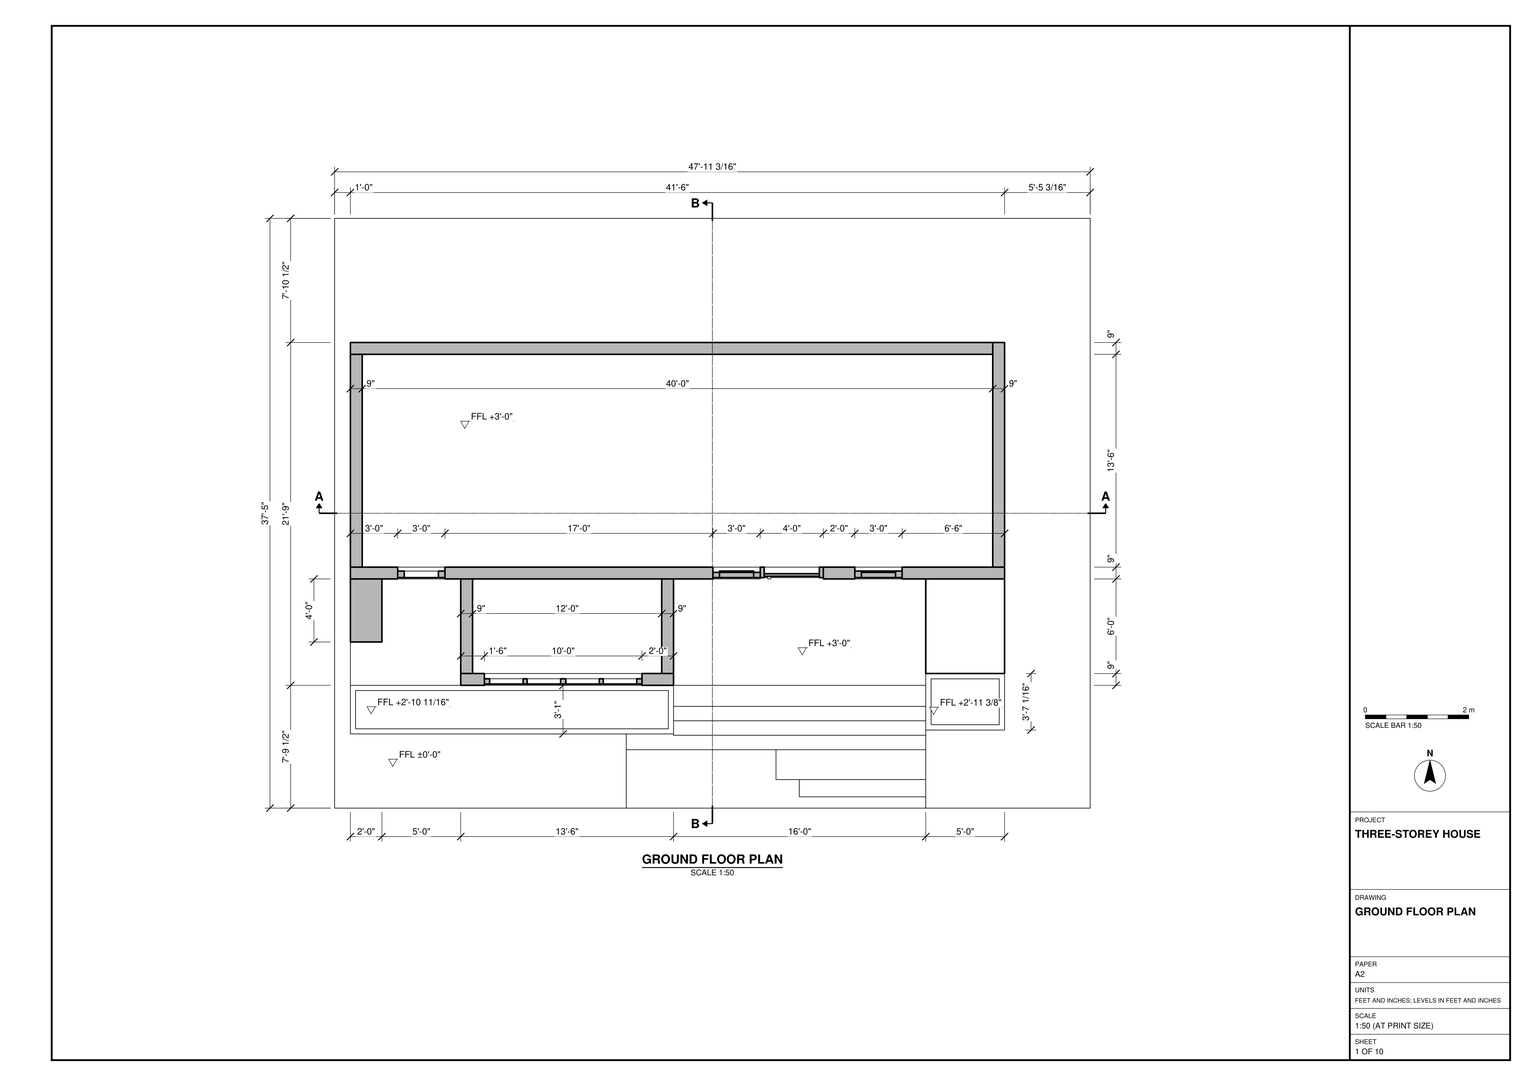
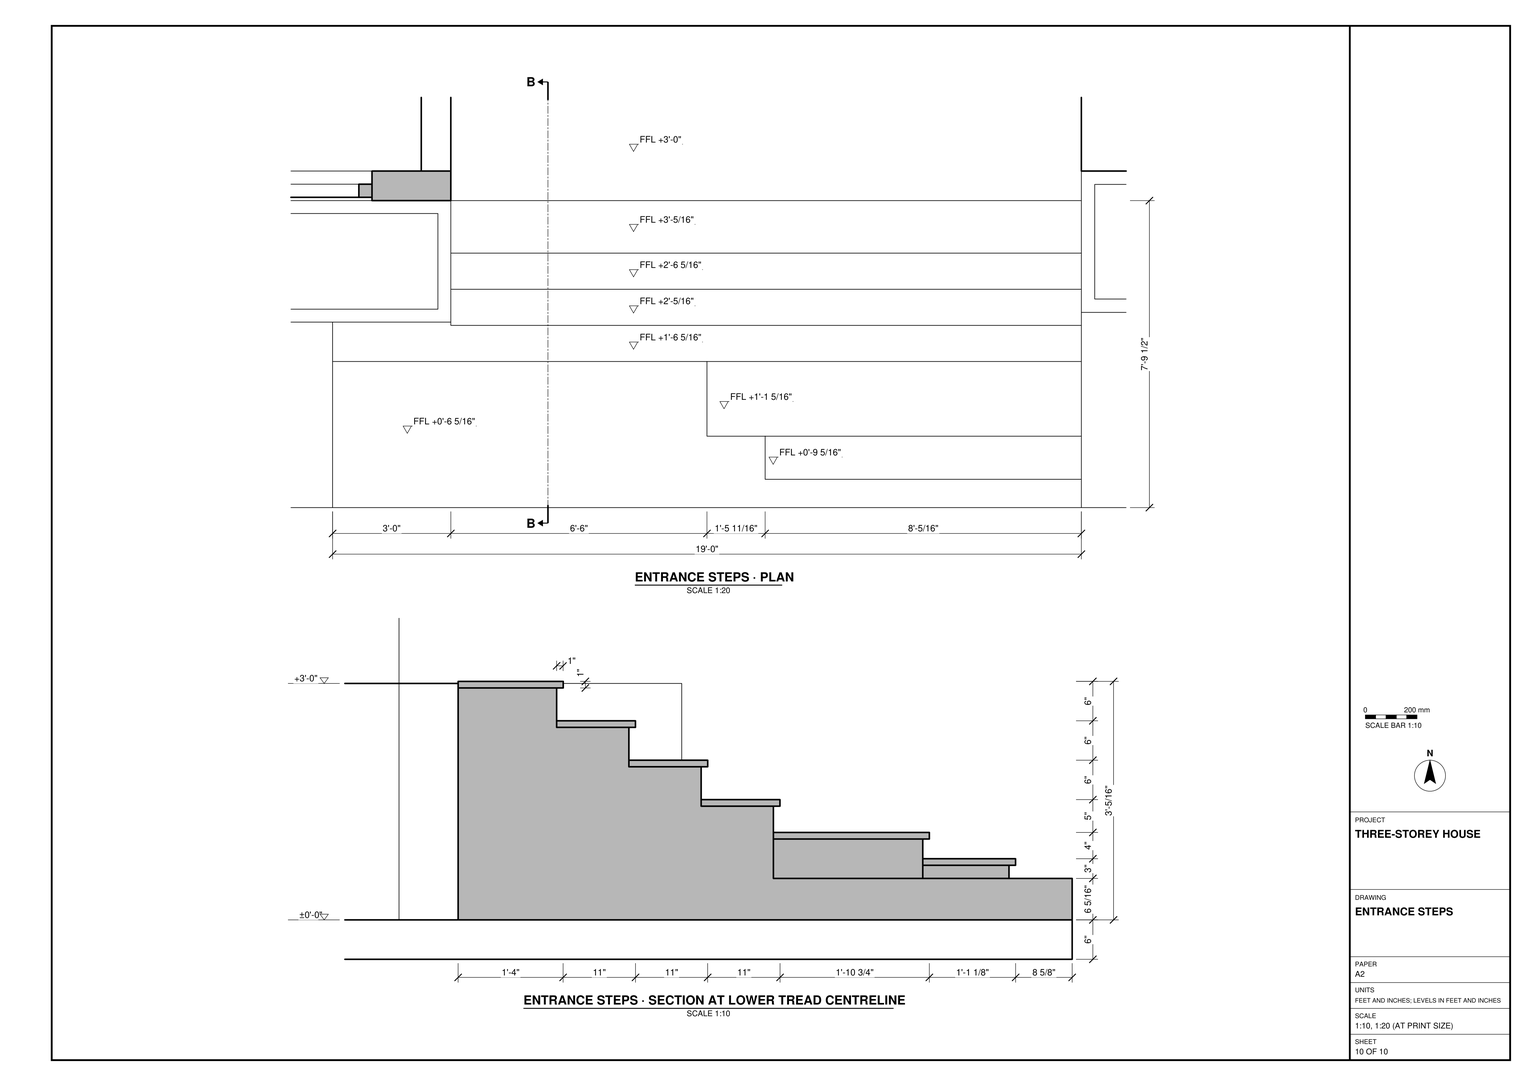
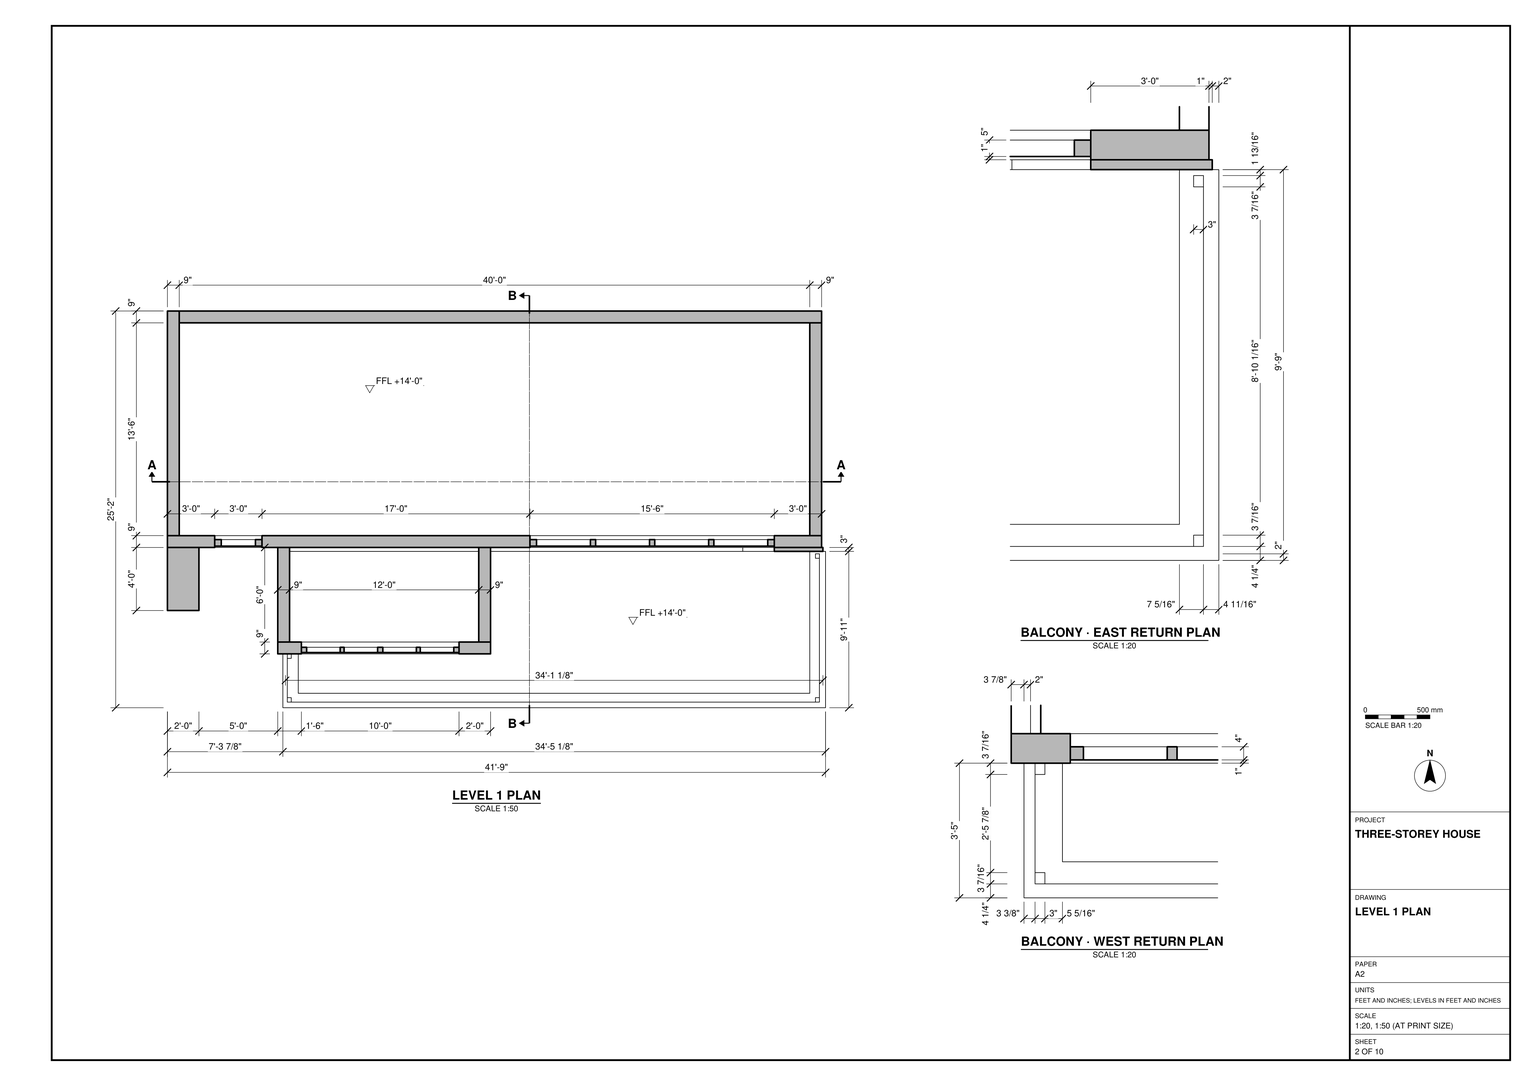
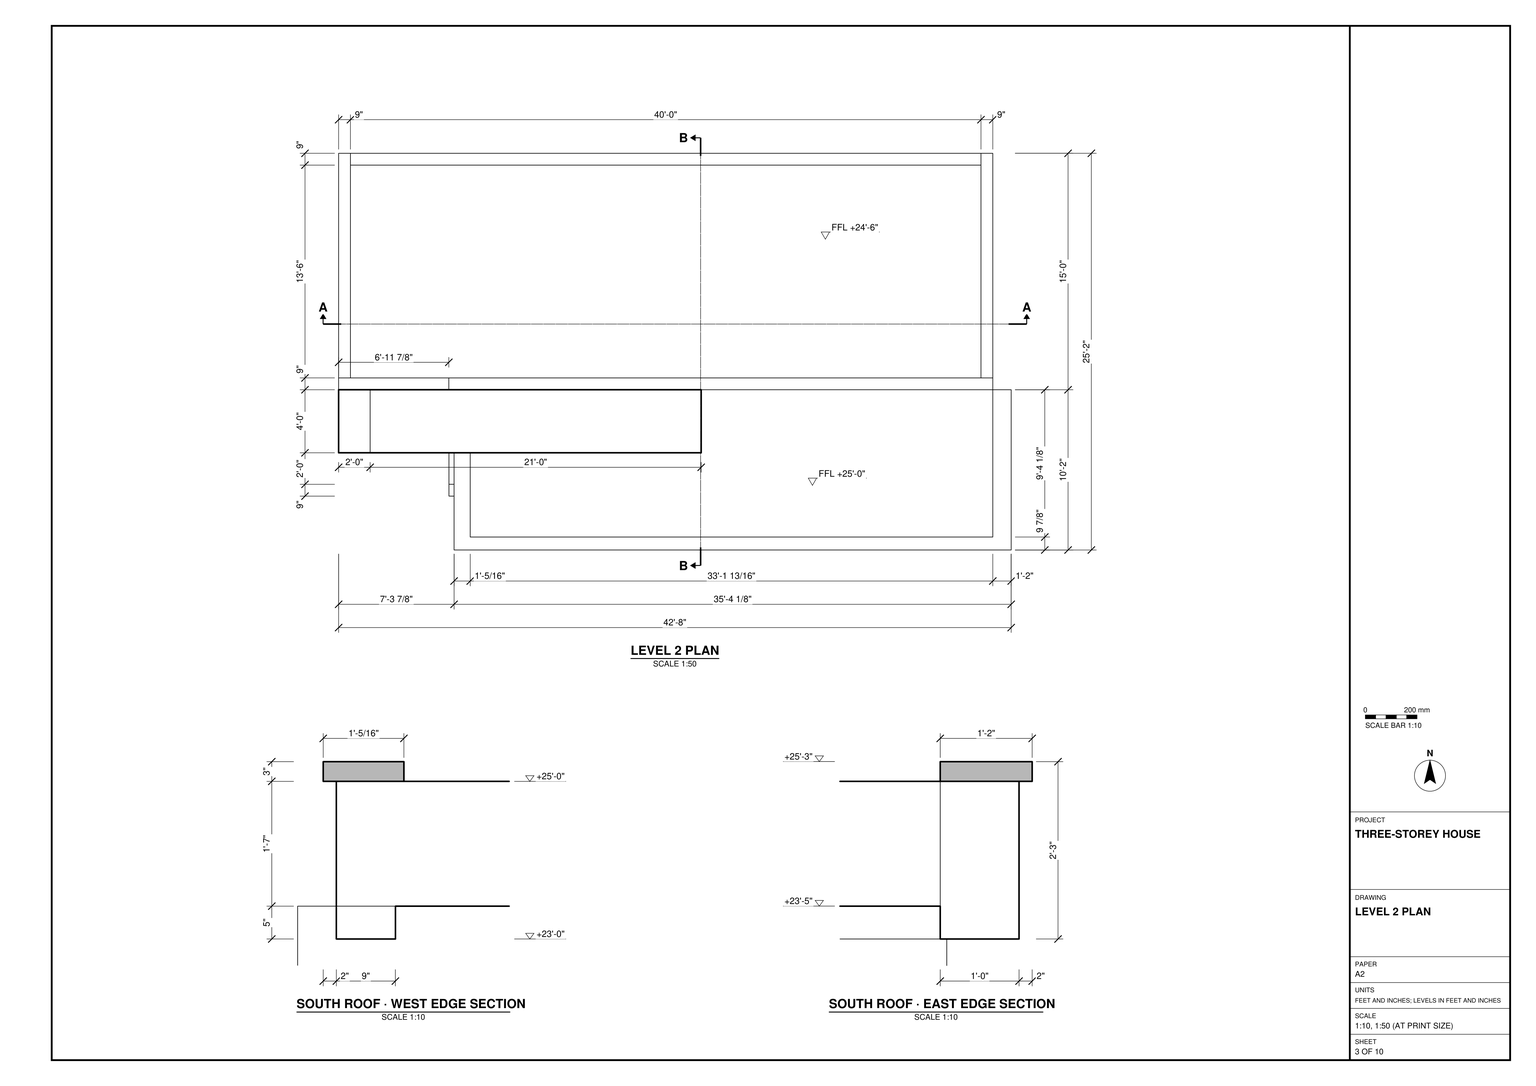
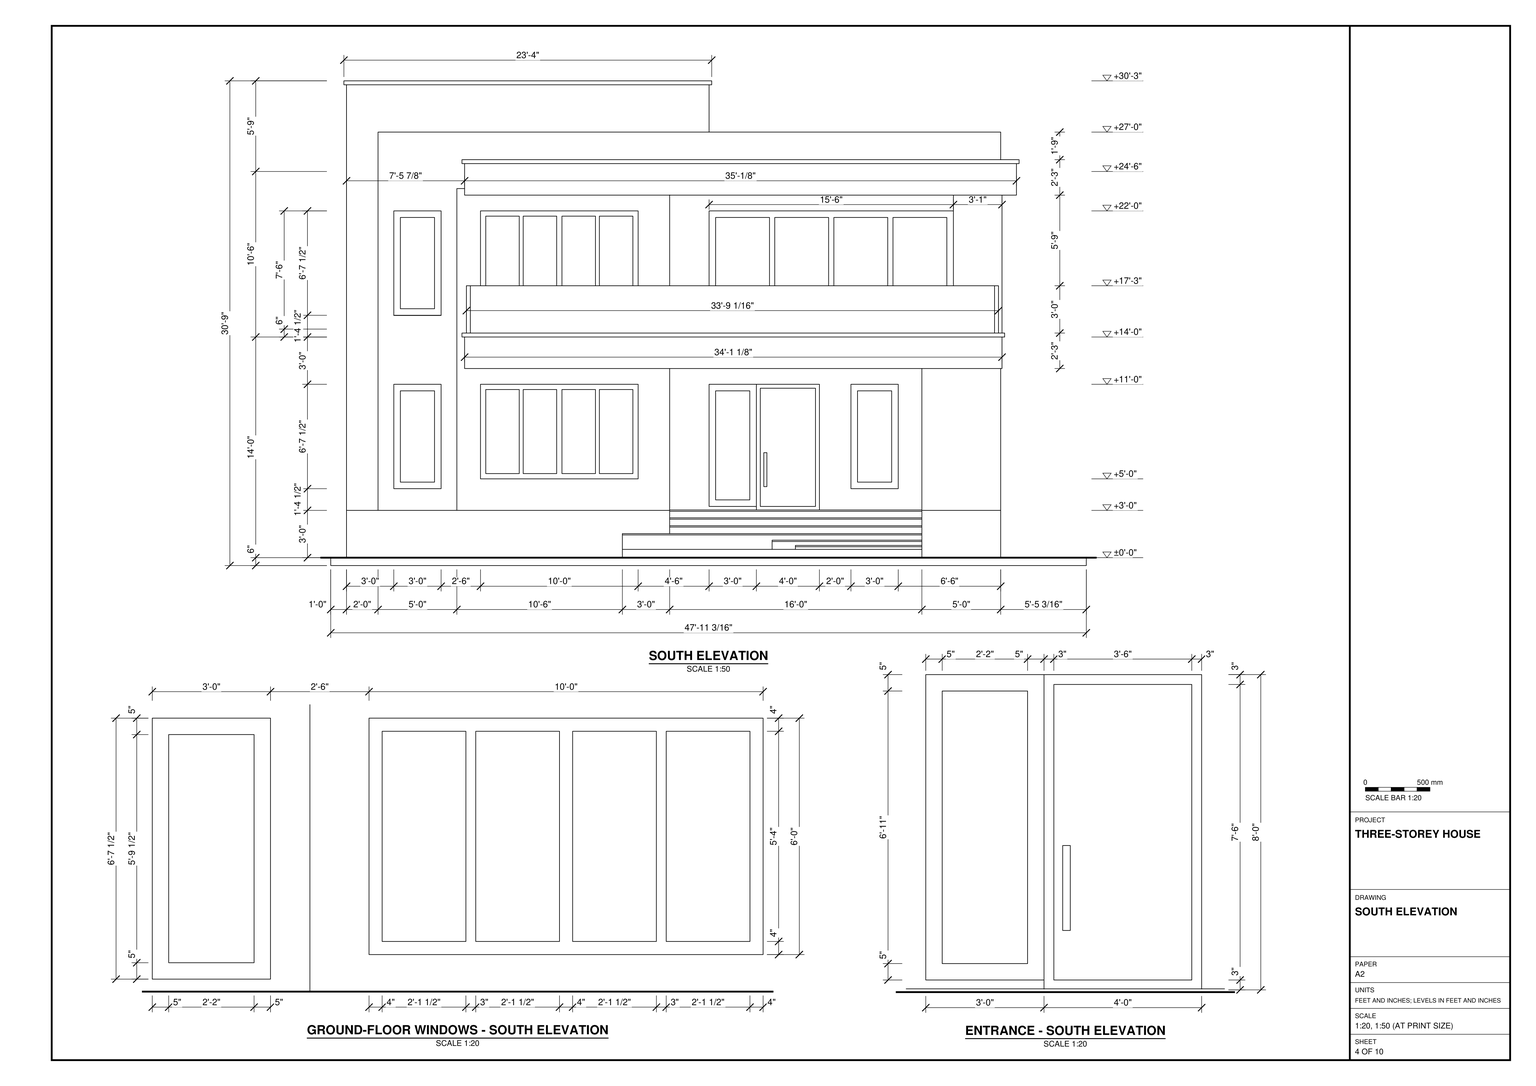
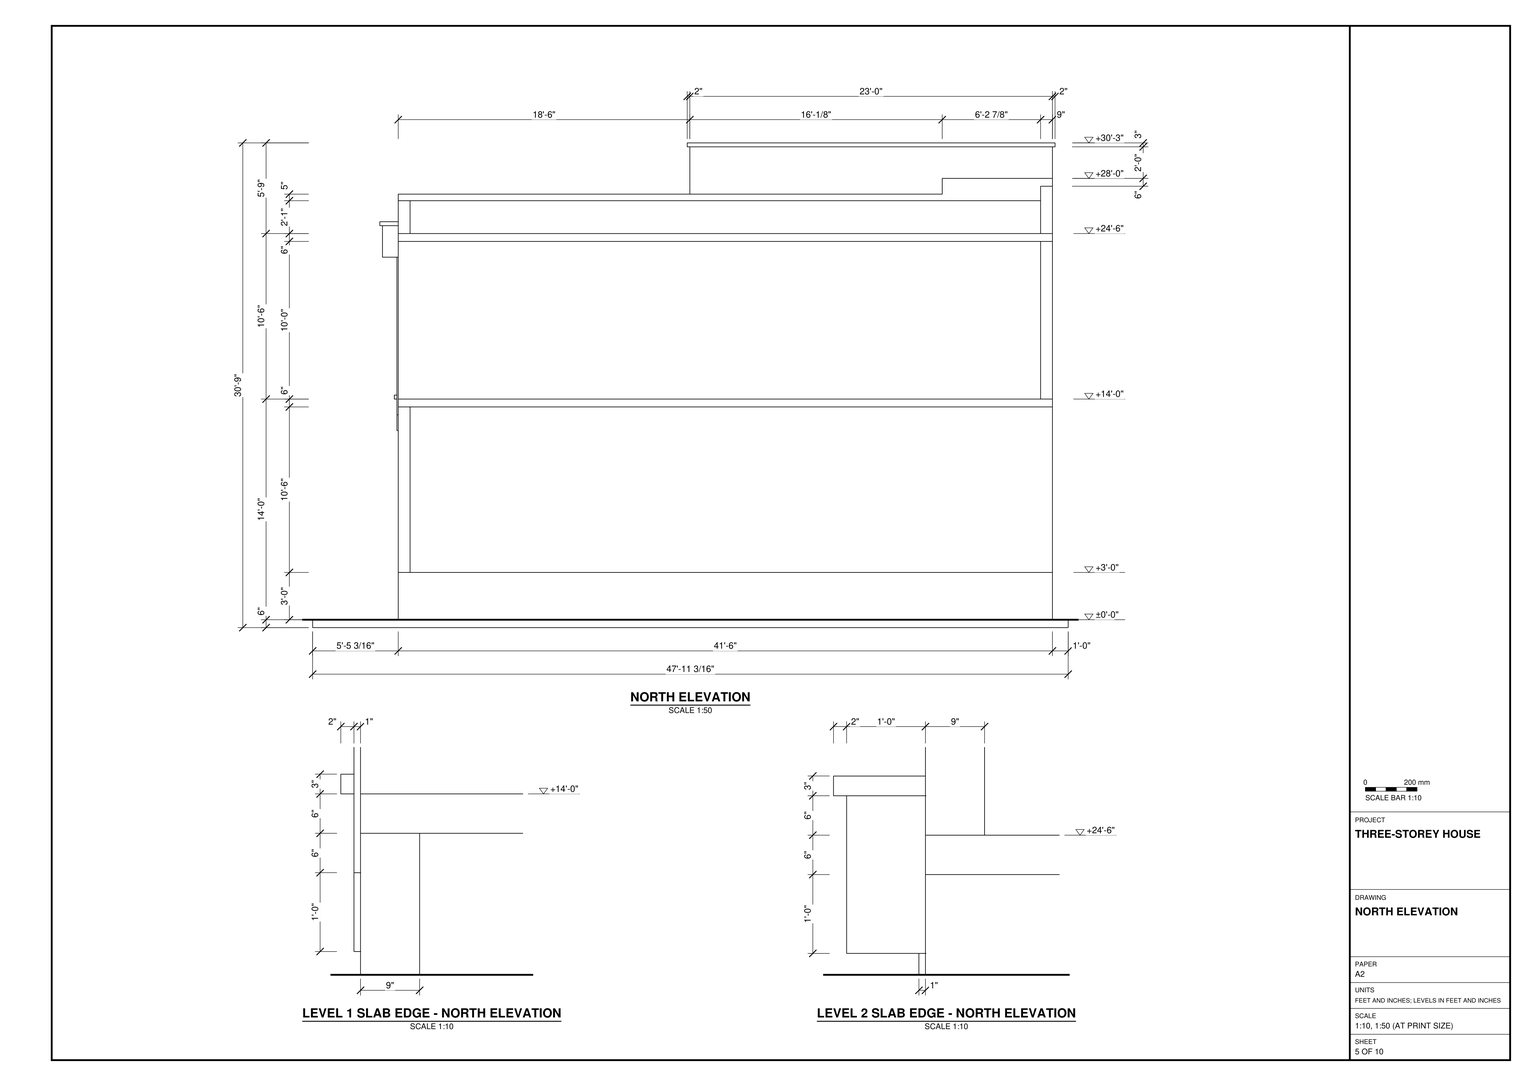
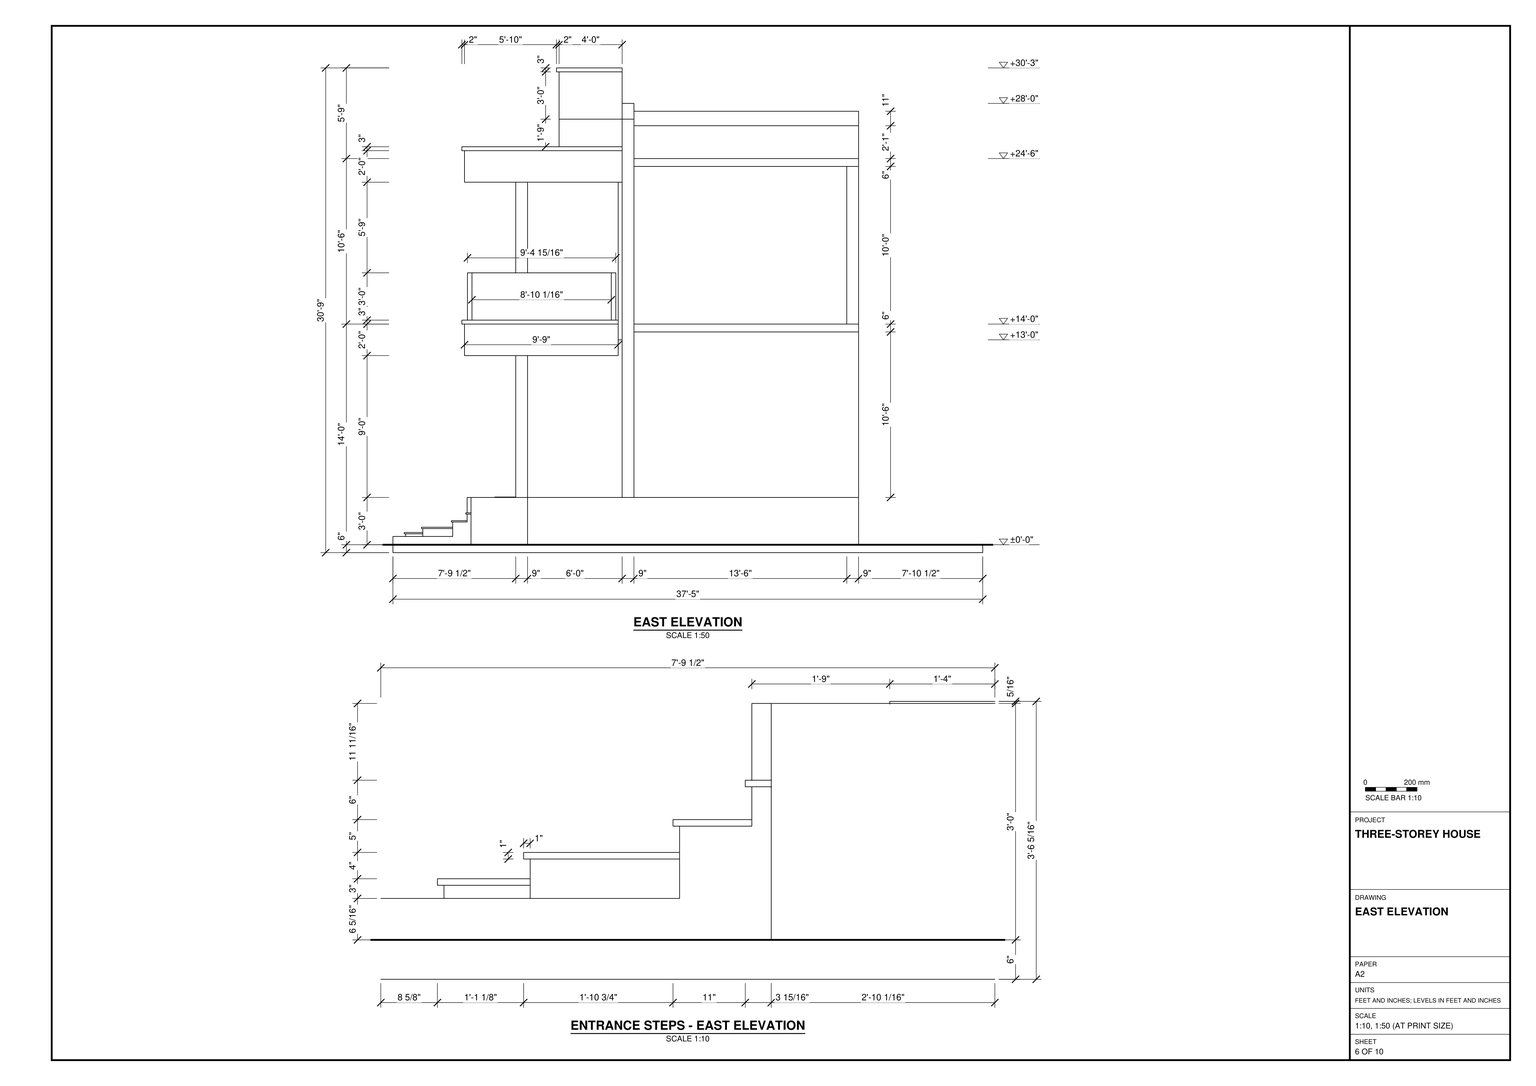
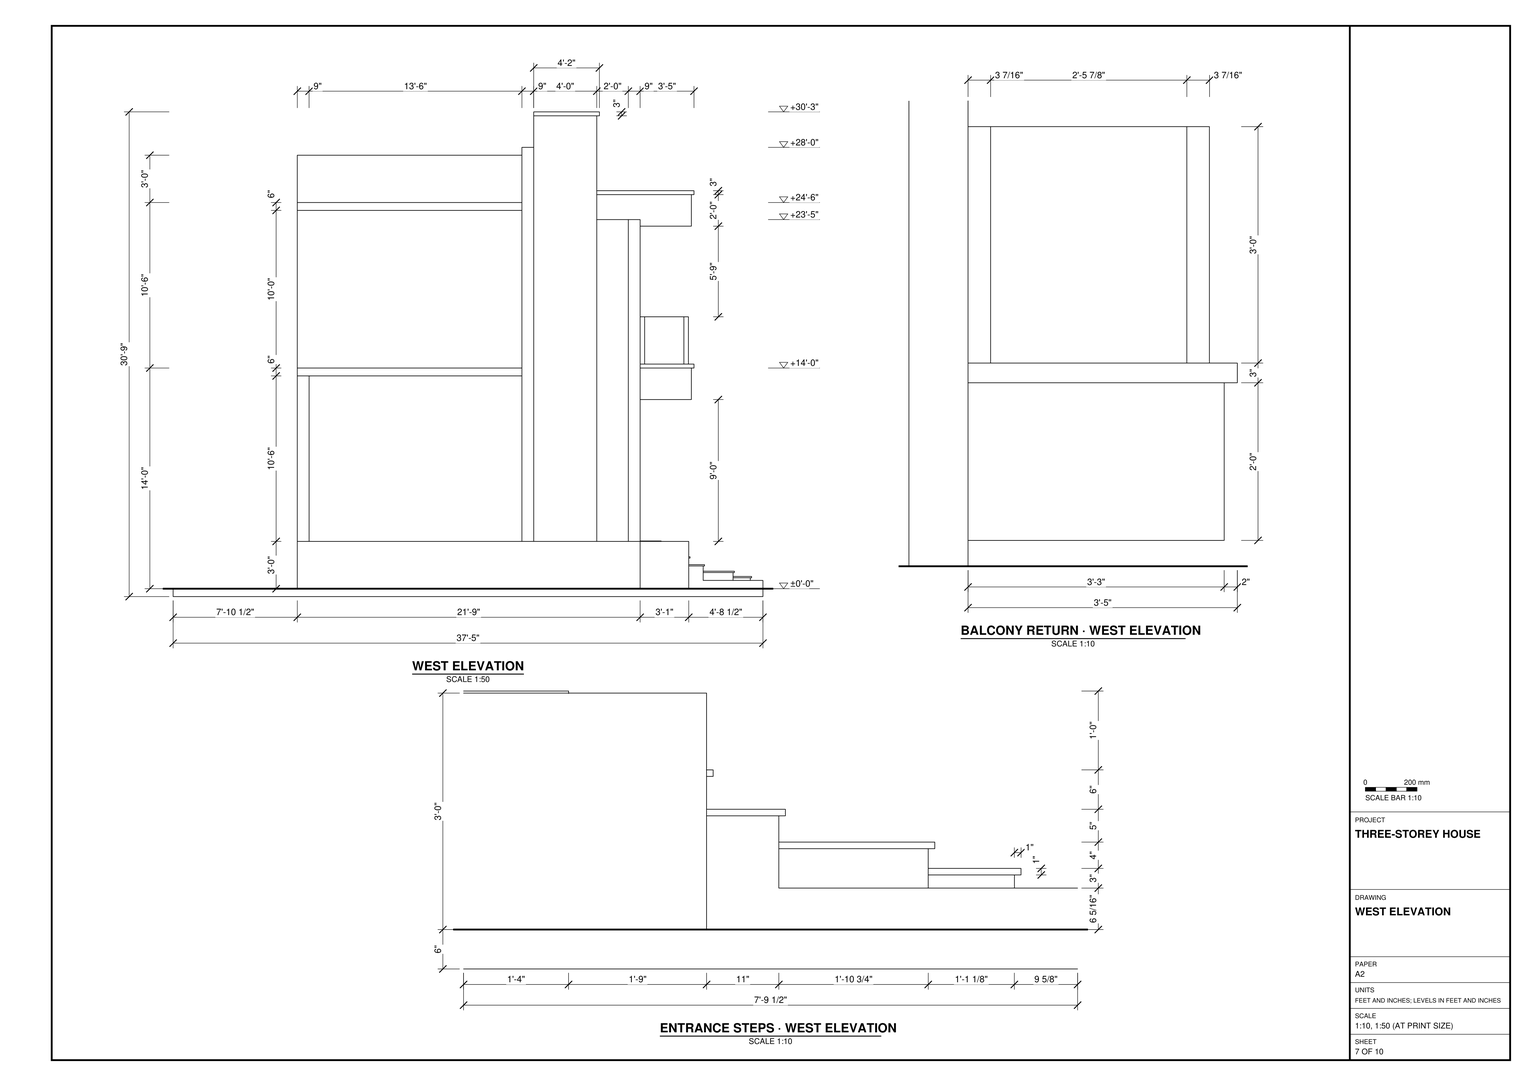
Build the house in SketchUp from task_files/diagram_01.pdf. Work in feet and inches. Including the site base, the model must measure 47'-11 3/16" across the frontage, 37'-5" from front to back and 30'-9" in overall height. Use the reference levels ±0'-0", +14'-0" and +24'-6". Distinguish the site datum from the raised ground floor and entrance landing at +3'-0".

Lay out the rectangular main enclosure with the 9" walls shown in plan. Form the projecting front bay to the left of the entrance and align its ground-floor and upper walls. Place the door and window units in their drawn openings, including the divided glazing across the bay. Model the entrance steps from both the enlarged plan and the section: the lower treads are offset rather than a continuation of the full-width upper flight. At +14'-0", carry the balcony past the projecting bay and follow the separate details for its east and west returns. Complete the floor slabs, upper enclosure and roof to the profiles shown. Include built-in joinery and main furniture where shown. Any decor and loose items shown may be suitable library components.

Keep walls, slabs, roof and each furniture or joinery piece in separate groups or components, and use components for repeated parts. Save one SketchUp model as output_files/three_storey_house_front_balcony_and_entrance_steps.skp.

# SketchUp Ruby script. Lengths in inches.
U = 1.inch
M = Sketchup.active_model
def pt(a) = Geom::Point3d.new(a.map { |v| v * U })
def face(e, loops, mat)
  f = e.add_face(loops[0].map { |a| pt(a) })
  loops[1..].each { |l| e.add_face(l.map { |a| pt(a) }).erase! }
  f.material = f.back_material = mat if mat
  f
end
# faces: each face lists its corners as indices into pts; further lists are holes
def faces(e, pts, list, mat = nil) = list.each { |f| face(e, (f[0].is_a?(Array) ? f : [f]).map { |l| l.map { |i| pts[i] } }, mat) }
# xy, xz, yz: faces in a plane at the given z, y or x. An outline is a flat list of corners, or four numbers for a rectangle; further outlines are holes
def ring(l) = l.size == 4 ? [[l[0], l[1]], [l[2], l[1]], [l[2], l[3]], [l[0], l[3]]] : l.each_slice(2).to_a
def flat(e, list, mat, &to3) = list.each { |f| face(e, (f[0].is_a?(Array) ? f : [f]).map { |l| ring(l).map { |u, v| to3.(u, v) } }, mat) }
def xy(e, z, list, mat = nil) = flat(e, list, mat) { |x, y| [x, y, z] }
def xz(e, y, list, mat = nil) = flat(e, list, mat) { |x, z| [x, y, z] }
def yz(e, x, list, mat = nil) = flat(e, list, mat) { |y, z| [x, y, z] }
def lines(e, pts, list) = list.each { |a, b| e.add_line(pt(pts[a]), pt(pts[b])) }
# prism: a flat outline (further loops are holes) pulled along v
def prism(e, loops, v, mat = nil)
  f = face(e, loops, mat); d = Geom::Vector3d.new(v.map { |x| x * U })
  f.pushpull(f.normal.samedirection?(d) ? d.length : -d.length)
end
def box(e, o, s, mat = nil) = prism(e, [[o, [o[0] + s[0], o[1], o[2]], [o[0] + s[0], o[1] + s[1], o[2]], [o[0], o[1] + s[1], o[2]]]], [0, 0, s[2]], mat)
def at(x, y, z, deg = 0) = Geom::Transformation.translation(pt([x, y, z])) * Geom::Transformation.rotation(ORIGIN, Z_AXIS, deg.degrees)
def axes(o, x, y, z) = Geom::Transformation.new([*x, 0, *y, 0, *z, 0, *pt(o).to_a, 1])
def part(name) = M.definitions.add(name)
# library, detail: a bought-in or finely detailed component or shape, given as its bounding box
def library(name, o, s) = part(name).tap { |d| box(d.entities, o, s) }
def detail(e, o, s) = box(e.add_group.entities, o, s)
def put(e, d, t, mat = nil) = e.add_instance(d, t).tap { |i| i.material = mat if mat }
def group(e, t, mat = nil) = e.add_group.tap { |g| g.transformation = t; g.material = mat if mat }.entities
root = M.entities
M.materials.add("[Aluminum]").color = [179, 179, 179]
M.materials.add("[Blinds Cloth Horizontal]").color = [145, 84, 40]
M.materials.add("[Color M07]").color = [58, 58, 58]
M.materials.add("[Color M09]").color = [0, 0, 0]
M.materials.add("[Grass Dark Green]").color = [106, 157, 55]
M.materials.add("[Stone Sandstone Ashlar Light]").color = [209, 180, 129]
M.materials.add("[Translucent Glass Blue]").color = [100, 149, 237]
M.materials["[Translucent Glass Blue]"].alpha = 0.5
M.materials.add("[Translucent Glass Gray]").color = [204, 204, 204]
M.materials["[Translucent Glass Gray]"].alpha = 0.5
M.materials.add("[Window Covering 02]").color = [198, 168, 91]
M.materials.add("[Wood Bamboo]").color = [177, 105, 43]
M.materials.add("[Wood Veneer 01]").color = [120, 70, 37]
c1 = part("Group\#19")
prism(c1.entities,[[[0,5,79.48],[36,5,79.48],[36,5,0],[0,5,0]],[[5,5,5],[31,5,5],[31,5,74.48],[5,5,74.48]]],[0,-5,0])
c2 = part("Group\#51")
box(c2.entities,[0,2,0],[3,3.4375,36])
g1 = group(root,at(8.16,0,0))
box(g1,[-8.16,0,0],[575.16,449,6])
g2 = group(root,at(90,114.49,6))
prism(g2,[[[-78,-21,0],[-78,240,0],[420,240,0],[420,-12,0],[360,-12,0],[360,-21,0]]],[0,0,36])
g3 = group(root,at(90,174.49,42))
prism(g3,[[[234,9,0],[-78,9,0],[-78,9,300],[5.89,9,300],[5.89,9,288],[420,9,288],[420,9,0],[282,9,0],[282,9,96],[234,9,96],[198,9,96],[198,9,3],[234,9,3]],[[198,9,228],[198,9,132],[384,9,132],[384,9,228]],[[-6,9,228],[-42,9,228],[-42,9,148.37],[-6,9,148.37]],[[306,9,96],[306,9,16.52],[342,9,16.52],[342,9,96]],[[-6,9,96],[-42,9,96],[-42,9,16.52],[-6,9,16.52]]],[0,-9,0])
g4 = group(root,at(450,54.49,42),"[Stone Sandstone Ashlar Light]")
box(g4,[0,48,0],[60,72,120])
g5 = group(root,at(396,175.49,58.52),"[Color M09]")
prism(g5,[[[0,5,79.48],[36,5,79.48],[36,5,0],[0,5,0]],[[5,5,5],[31,5,5],[31,5,74.48],[5,5,74.48]]],[0,-5,0])
g6 = group(root,at(401,175.49,63.52),"[Translucent Glass Gray]")
xz(g6,0,[[0,0,26,69.48]])
g7 = group(root,at(324,175.49,42),"[Wood Bamboo]")
prism(g7,[[[0,8,0],[0,8,96],[48,8,96],[48,8,0]],[[45,8,93],[3,8,93],[3,8,3],[45,8,3]]],[0,-8,0])
g8 = group(root,at(327,176.49,45),"[Wood Bamboo]")
box(g8,[0,0,0],[42,2,90])
g9 = group(root,at(288,175.49,45),"[Color M09]")
prism(g9,[[[0,4,93],[36,4,93],[36,4,0],[0,4,0]],[[5,4,88],[5,4,5],[31,4,5],[31,4,88]]],[0,-4,0])
g10 = group(root,at(293,179.49,50),"[Wood Bamboo]")
box(g10,[0,0,0],[26,1,83])
g11 = group(root,at(57,93.49,42))
prism(g11,[[[201,9,0],[39,9,0],[39,9,245],[201,9,245]],[[57,9,228],[57,9,138],[177,9,138],[177,9,228]],[[177,9,24],[177,9,96],[57,9,96],[57,9,24]]],[0,-9,0])
g12 = group(root,at(249,63.49,42))
box(g12,[0,39,0],[9,72,120])
g13 = group(root,at(96,63.49,42))
box(g13,[0,39,0],[9,72,245])
put(root,c1,at(48,175.49,58.52),"[Color M09]")
g14 = group(root,at(53,175.49,63.52),"[Translucent Glass Blue]")
xz(g14,0,[[0,0,26,69.48]])
g15 = group(root,at(114,94.49,66),"[Translucent Glass Blue]")
g16 = group(g15,at(62,0,4))
xz(g16,0,[[0,0,25.5,64]])
g17 = group(g15,at(32.5,0,4))
xz(g17,0,[[0,0,25.5,64]])
g18 = group(g15,at(90.5,0,4))
xz(g18,0,[[0,0,25.5,64]])
g19 = group(g15,at(4,0,4))
xz(g19,0,[[0,0,25.5,64]])
g20 = group(g15,at(0,0,0),"[Color M09]")
prism(g20,[[[120,4,0],[0,4,0],[0,4,72],[120,4,72]],[[29.5,4,4],[29.5,4,68],[4,4,68],[4,4,4]],[[90.5,4,68],[90.5,4,4],[116,4,4],[116,4,68]],[[32.5,4,4],[58,4,4],[58,4,68],[32.5,4,68]],[[62,4,4],[87.5,4,4],[87.5,4,68],[62,4,68]]],[0,-4,0])
g21 = group(root,at(12,126.49,42))
prism(g21,[[[0,48,324],[276,48,324],[276,48,288],[24,48,288],[24,48,0],[0,48,0]]],[0,-48,0])
g22 = group(root,at(12,183.49,42))
box(g22,[0,0,0],[9,162,126])
g23 = group(root,at(12,345.49,42))
box(g23,[0,0,0],[489,9,126])
g24 = group(root,at(501,183.49,42))
box(g24,[0,0,0],[9,171,126])
g25 = group(root,at(12,174.49,168))
box(g25,[0,9,0],[498,171,6])
g26 = group(root,at(96,78.49,150))
xy(g26,0,[[[5.89,-24,415,93],[16,-12,403,84]]])
xy(g26,5,[[16,-12,403,84]],"[Blinds Cloth Horizontal]")
xy(g26,24,[[5.89,-24,415,93]])
xz(g26,-24,[[5.89,0,415,24]])
xz(g26,-12,[[16,0,403,5]])
xz(g26,84,[[16,0,403,5]])
xz(g26,93,[[5.89,0,415,24]])
yz(g26,5.89,[[-24,0,93,24]])
yz(g26,16,[[-12,0,84,5]])
yz(g26,403,[[-12,0,84,5]])
yz(g26,415,[[-24,0,93,24]])
g27 = group(root,at(288,175.49,174),"[Color M09]")
prism(g27,[[[0,5,0],[0,5,96],[186,5,96],[186,5,0]],[[140,5,91],[140,5,5],[181,5,5],[181,5,91]],[[5,5,5],[46,5,5],[46,5,91],[5,5,91]],[[50,5,5],[91,5,5],[91,5,91],[50,5,91]],[[95,5,5],[136,5,5],[136,5,91],[95,5,91]]],[0,-5,0])
g28 = group(root,at(428,175.49,179),"[Translucent Glass Blue]")
xz(g28,0,[[0,0,41,86]])
g29 = group(root,at(383,175.49,179),"[Translucent Glass Blue]")
xz(g29,0,[[0,0,41,86]])
g30 = group(root,at(338,175.49,179),"[Translucent Glass Blue]")
xz(g30,0,[[0,0,41,86]])
g31 = group(root,at(293,175.49,179),"[Translucent Glass Blue]")
xz(g31,0,[[0,0,41,86]])
g32 = group(root,at(249,102.49,174))
box(g32,[0,0,0],[9,72,113])
g33 = group(root,at(114,94.49,180),"[Color M09]")
prism(g33,[[[0,4,0],[0,4,90],[120,4,90],[120,4,0]],[[90.5,4,86],[90.5,4,4],[116,4,4],[116,4,86]],[[32.5,4,86],[32.5,4,4],[58,4,4],[58,4,86]],[[87.5,4,86],[62,4,86],[62,4,4],[87.5,4,4]],[[4,4,4],[29.5,4,4],[29.5,4,86],[4,4,86]]],[0,-4,0])
g34 = group(root,at(204.5,94.49,184),"[Translucent Glass Blue]")
xz(g34,0,[[0,0,25.5,82]])
g35 = group(root,at(176,94.49,184),"[Translucent Glass Blue]")
xz(g35,0,[[0,0,25.5,82]])
g36 = group(root,at(146.5,94.49,184),"[Translucent Glass Blue]")
xz(g36,0,[[0,0,25.5,82]])
g37 = group(root,at(118,94.49,184),"[Translucent Glass Blue]")
xz(g37,0,[[0,0,25.5,82]])
put(root,c1,at(48,175.49,190.52),"[Color M09]")
g38 = group(root,at(53,175.49,195.52),"[Translucent Glass Blue]")
xz(g38,0,[[0,0,26,69.48]])
g39 = group(root,at(95.89,54.49,282))
xy(g39,0,[[[6,0,426.11,120],[15,12,414.11,108]]])
xy(g39,5,[[15,12,414.11,108]],"[Blinds Cloth Horizontal]")
xy(g39,24,[[6,0,426.11,120]])
xz(g39,0,[[6,0,426.11,24]])
xz(g39,12,[[15,0,414.11,5]])
xz(g39,108,[[15,0,414.11,5]])
xz(g39,120,[[6,0,426.11,24]])
yz(g39,6,[[0,0,120,24]])
yz(g39,15,[[12,0,108,5]])
yz(g39,414.11,[[12,0,108,5]])
yz(g39,426.11,[[0,0,120,24]])
g40 = group(root,at(501,183.49,174))
box(g40,[0,0,0],[9,162,120])
g41 = group(root,at(12,183.49,174))
box(g41,[0,0,0],[9,171,120])
g42 = group(root,at(21,345.49,174))
box(g42,[0,0,0],[489,9,120])
g43 = group(root,at(12,183.49,294))
box(g43,[0,0,0],[498,171,6])
g44 = group(root,at(12,183.49,300))
box(g44,[0,0,0],[9,171,36])
g45 = group(root,at(501,183.49,300))
box(g45,[0,0,0],[9,171,25])
g46 = group(root,at(21,345.49,300))
box(g46,[0,0,0],[480,9,25])
g47 = group(root,at(101.89,54.49,174),"[Color M09]")
xy(g47,0,[[-2,-2,9.71,39],[9.71,-2,411.11,8.98],[399.11,8.98,411.11,117]])
xy(g47,3,[[-2,-2,411.11,-2,411.11,117,399.11,117,399.11,8.98,9.71,8.98,9.71,39,-2,39]])
xz(g47,-2,[[-2,0,411.11,3]])
xz(g47,8.98,[[9.71,0,399.11,3]])
xz(g47,39,[[-2,0,9.71,3]])
xz(g47,117,[[399.11,0,411.11,3]])
yz(g47,-2,[[-2,0,39,3]])
yz(g47,9.71,[[8.98,0,39,3]])
yz(g47,399.11,[[8.98,0,117,3]])
yz(g47,411.11,[[-2,0,117,3]])
g48 = group(root,at(101.89,54.49,306),"[Color M09]")
xy(g48,0,[[-2,-2,10.29,120],[10.29,-2,422.11,7.875],[408.11,7.875,422.11,120]])
xy(g48,3,[[-2,-2,422.11,-2,422.11,120,408.11,120,408.11,7.875,10.29,7.875,10.29,120,-2,120]])
xz(g48,-2,[[-2,0,422.11,3]])
xz(g48,7.875,[[10.29,0,408.11,3]])
xz(g48,120,[[-2,0,10.29,3],[408.11,0,422.11,3]])
yz(g48,-2,[[-2,0,120,3]])
yz(g48,10.29,[[7.875,0,120,3]])
yz(g48,408.11,[[7.875,0,120,3]])
yz(g48,422.11,[[-2,0,120,3]])
g49 = group(root,at(12,126.49,366),"[Color M09]")
box(g49,[-2,-2,0],[280,50,3])
put(root,c2,at(103.26,88.05,177),"[Aluminum]")
put(root,c2,at(103.26,54.74,177),"[Aluminum]")
put(root,c2,at(505.33,54.74,177),"[Aluminum]")
g50 = group(root,at(106.26,56.74,177),"[Translucent Glass Blue]")
xz(g50,0,[[0,0,399.0625,36]])
g51 = group(root,at(103.26,60.18,177))
yz(g51,0,[[0,0,29.875,36]])
g52 = group(root,at(258,38.49,12.3125))
xy(g52,-6.3125,[[-36,-38.49,-36,18,0,18,0,55,192,55,192,-38.49]])
xy(g52,0,[[-36,-38.49,192,7]])
xy(g52,11,[[-36,6,192,7],[-36,7,192,18]])
xy(g52,12,[[-36,6,192,18]])
xy(g52,17,[[0,17,192,18],[0,18,192,29]])
xy(g52,18,[[0,17,192,29]])
xy(g52,23,[[0,28,192,29],[0,29,192,40]])
xy(g52,24,[[0,28,192,40]])
xy(g52,29,[[0,39,192,40],[0,40,192,55]])
xy(g52,30,[[0,39,192,55]])
xz(g52,-38.49,[[-36,-6.3125,192,0]])
xz(g52,6,[[-36,11,192,12]])
xz(g52,7,[[-36,0,192,11]])
xz(g52,17,[[0,17,192,18]])
xz(g52,18,[[-36,-6.3125,0,11],[-36,11,0,12],[0,11,192,12],[0,12,192,17]])
xz(g52,28,[[0,23,192,24]])
xz(g52,29,[[0,17,192,18],[0,18,192,23]])
xz(g52,39,[[0,29,192,30]])
xz(g52,40,[[0,23,192,24],[0,24,192,29]])
xz(g52,55,[[0,-6.3125,192,29],[0,29,192,30]])
yz(g52,-36,[[-38.49,-6.3125,-38.49,0,7,0,7,11,18,11,18,-6.3125],[6,11,18,12]])
yz(g52,0,[[18,-6.3125,18,17,29,17,29,23,40,23,40,29,55,29,55,-6.3125],[17,17,29,18],[28,23,40,24],[39,29,55,30]])
yz(g52,192,[[-38.49,-6.3125,55,-6.3125,55,29,40,29,40,23,29,23,29,17,18,17,18,11,7,11,7,0,-38.49,0],[6,11,18,12],[17,17,29,18],[28,23,40,24],[39,29,55,30]])
g53 = group(root,at(335.99,22.74,15.3125))
xy(g53,-3,[[0,0,114.01,22.74]])
xy(g53,3,[[0,-1,114.01,0],[0,0,114.01,22.74]])
xy(g53,4,[[0,-1,114.01,22.74]])
xz(g53,-1,[[0,3,114.01,4]])
xz(g53,0,[[0,-3,114.01,3]])
xz(g53,22.74,[[0,-3,114.01,3],[0,3,114.01,4]])
yz(g53,0,[[0,-3,22.74,3],[-1,3,22.74,4]])
yz(g53,114.01,[[0,-3,22.74,3],[-1,3,22.74,4]])
g54 = group(root,at(353.71,9.62,12.3125))
xy(g54,0,[[0,0,96.29,13.125]])
xy(g54,2,[[0,-1,96.29,0],[0,0,96.29,13.125]])
xy(g54,3,[[0,-1,96.29,13.125]])
xz(g54,-1,[[0,2,96.29,3]])
xz(g54,0,[[0,0,96.29,2]])
xz(g54,13.125,[[0,0,96.29,2],[0,2,96.29,3]])
yz(g54,0,[[0,0,13.125,2],[-1,2,13.125,3]])
yz(g54,96.29,[[0,0,13.125,2],[-1,2,13.125,3]])
g55 = group(root,at(12,56.49,6),"[Color M07]")
xy(g55,0,[[0,0,246,37]])
xy(g55,34.6875,[[3.93,3.93,242.07,33.07]],"[Grass Dark Green]")
xy(g55,36,[[[0,0,246,37],[3.93,3.93,242.07,33.07]]])
xz(g55,0,[[0,0,246,36]])
xz(g55,3.93,[[3.93,34.6875,242.07,36]])
xz(g55,33.07,[[3.93,34.6875,242.07,36]])
xz(g55,37,[[0,0,246,36]])
yz(g55,0,[[0,0,37,36]])
yz(g55,3.93,[[3.93,34.6875,33.07,36]])
yz(g55,242.07,[[3.93,34.6875,33.07,36]])
yz(g55,246,[[0,0,37,36]])
g56 = group(root,at(450,59.44,6),"[Window Covering 02]")
xy(g56,0,[[0,0,60,43.05]])
xy(g56,35.375,[[4.07,4.07,55.93,38.98]],"[Grass Dark Green]")
xy(g56,36,[[[0,0,60,43.05],[4.07,4.07,55.93,38.98]]])
xz(g56,0,[[0,0,60,36]])
xz(g56,4.07,[[4.07,35.375,55.93,36]])
xz(g56,38.98,[[4.07,35.375,55.93,36]])
xz(g56,43.05,[[0,0,60,36]])
yz(g56,0,[[0,0,43.05,36]])
yz(g56,4.07,[[4.07,35.375,38.98,36]])
yz(g56,55.93,[[4.07,35.375,38.98,36]])
yz(g56,60,[[0,0,43.05,36]])
g57 = group(root,at(329.69,174.49,60.08),"[Wood Veneer 01]")
box(g57,[0,0,0],[2.3125,2,25.875])
g58 = group(root,at(293,175.49,50),"[Translucent Glass Gray]")
xz(g58,0,[[0,0,26,83]])
g59 = group(root,at(474,171.49,162),"[Window Covering 02]")
box(g59,[0,0,0],[37,3,120])
put(root,c2,at(505.33,164.24,177),"[Aluminum]")
g60 = group(root,at(508.33,60.18,177),"[Translucent Glass Blue]")
yz(g60,0,[[0,0,106.0625,36]])
g61 = group(root,at(401,179.49,63.52),"[Wood Bamboo]")
box(g61,[0,0,0],[26,1,69.48])
